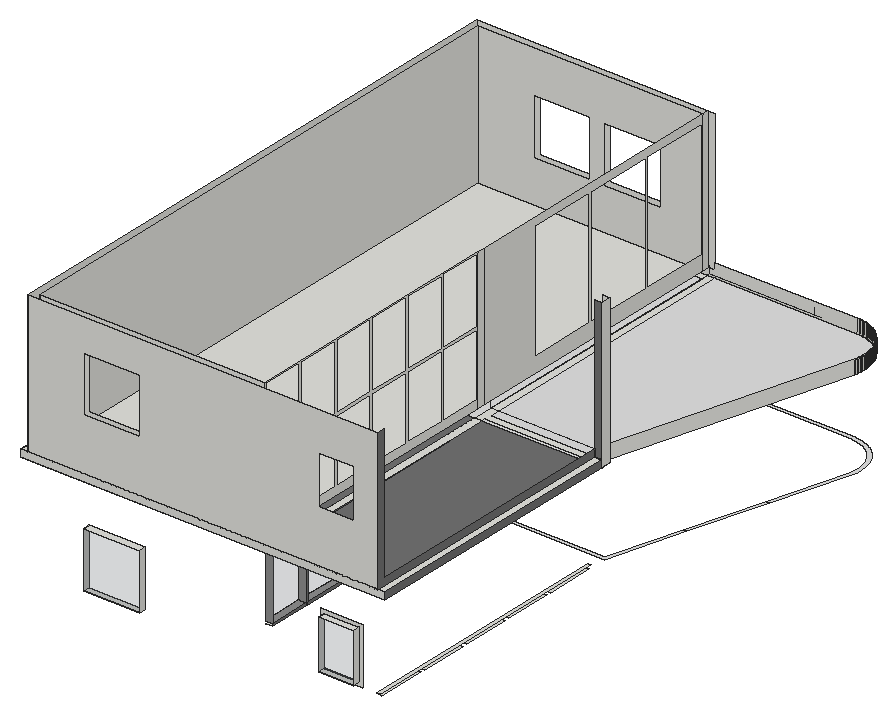
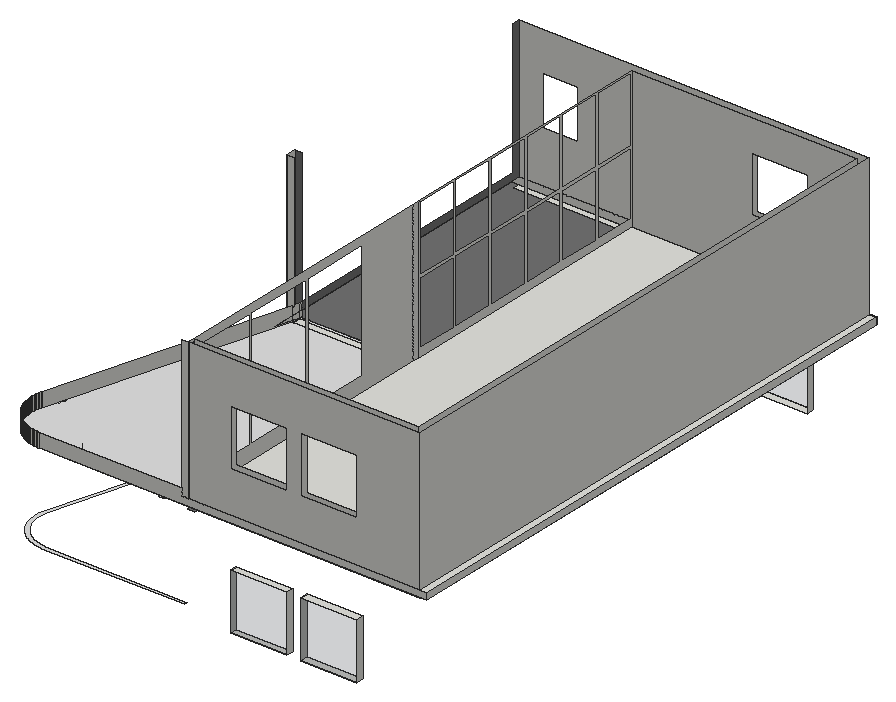
# SketchUp Ruby script. Lengths in inches.
U = 1.inch
M = Sketchup.active_model
def pt(a) = Geom::Point3d.new(a.map { |v| v * U })
def face(e, loops, mat)
  f = e.add_face(loops[0].map { |a| pt(a) })
  loops[1..].each { |l| e.add_face(l.map { |a| pt(a) }).erase! }
  f.material = f.back_material = mat if mat
  f
end
# faces: each face lists its corners as indices into pts; further lists are holes
def faces(e, pts, list, mat = nil) = list.each { |f| face(e, (f[0].is_a?(Array) ? f : [f]).map { |l| l.map { |i| pts[i] } }, mat) }
# xy, xz, yz: faces in a plane at the given z, y or x. An outline is a flat list of corners, or four numbers for a rectangle; further outlines are holes
def ring(l) = l.size == 4 ? [[l[0], l[1]], [l[2], l[1]], [l[2], l[3]], [l[0], l[3]]] : l.each_slice(2).to_a
def flat(e, list, mat, &to3) = list.each { |f| face(e, (f[0].is_a?(Array) ? f : [f]).map { |l| ring(l).map { |u, v| to3.(u, v) } }, mat) }
def xy(e, z, list, mat = nil) = flat(e, list, mat) { |x, y| [x, y, z] }
def xz(e, y, list, mat = nil) = flat(e, list, mat) { |x, z| [x, y, z] }
def yz(e, x, list, mat = nil) = flat(e, list, mat) { |y, z| [x, y, z] }
def lines(e, pts, list) = list.each { |a, b| e.add_line(pt(pts[a]), pt(pts[b])) }
# prism: a flat outline (further loops are holes) pulled along v
def prism(e, loops, v, mat = nil)
  f = face(e, loops, mat); d = Geom::Vector3d.new(v.map { |x| x * U })
  f.pushpull(f.normal.samedirection?(d) ? d.length : -d.length)
end
def box(e, o, s, mat = nil) = prism(e, [[o, [o[0] + s[0], o[1], o[2]], [o[0] + s[0], o[1] + s[1], o[2]], [o[0], o[1] + s[1], o[2]]]], [0, 0, s[2]], mat)
def at(x, y, z, deg = 0) = Geom::Transformation.translation(pt([x, y, z])) * Geom::Transformation.rotation(ORIGIN, Z_AXIS, deg.degrees)
def axes(o, x, y, z) = Geom::Transformation.new([*x, 0, *y, 0, *z, 0, *pt(o).to_a, 1])
def part(name) = M.definitions.add(name)
# library, detail: a bought-in or finely detailed component or shape, given as its bounding box
def library(name, o, s) = part(name).tap { |d| box(d.entities, o, s) }
def detail(e, o, s) = box(e.add_group.entities, o, s)
def put(e, d, t, mat = nil) = e.add_instance(d, t).tap { |i| i.material = mat if mat }
def group(e, t, mat = nil) = e.add_group.tap { |g| g.transformation = t; g.material = mat if mat }.entities
root = M.entities
M.materials.add("Glass_Basic_01").color = [105, 113, 122]
M.materials["Glass_Basic_01"].alpha = 0.25
M.materials.add("M01_Silver_Fog").color = [224, 224, 224]
M.materials.add("M04_Stone_Frost").color = [142, 142, 142]
M.materials.add("M06_Steel_Smoke").color = [114, 114, 114]
xy(root,300,[[54,0,102,6],[60,474,108,480],[120,474,168,480]])
xy(root,304,[[300,8,303,49],[300,53,303,94],[300,98,303,139],[300,143,303,184],[300,188,303,229]])
xy(root,306,[[300,6,303,231]])
xy(root,306,[[213,243,305.51,243,324.34,307.35,321.22,307.35,306,255.36,303.26,246,216,246,216,287.79,213,287.79],[321.22,307.35,324.34,307.35,343.2,371.78,340.07,371.78],[340.07,371.78,343.2,371.78,362.06,436.22,362.32,437.22,362.58,438.42,362.79,439.63,362.96,440.85,363.08,442.08,363.16,443.31,363.1875,444.54,363.17,445.77,363.1,447,362.99,448.22,362.83,449.44,362.63,450.66,362.38,451.86,362.08,453.06,361.74,454.24,361.35,455.41,360.92,456.5625,360.45,457.7,359.93,458.82,359.37,459.91,358.77,460.99,358.13,462.03,358.13,462.04,357.45,463.0625,356.73,464.0625,355.97,465.03,355.18,465.98,355.17,465.98,354.35,466.89,353.49,467.76,352.59,468.61,351.67,469.42,350.71,470.19,349.72,470.93,348.71,471.63,347.67,472.29,346.61,472.91,345.52,473.49,344.41,474.03,343.29,474.52,342.14,474.97,340.98,475.38,339.8,475.75,338.61,476.0625,337.41,476.34,336.2,476.5625,334.99,476.74,333.76,476.88,332.53,476.97,331.5,477,210,477,210,474,331.45,474,332.38,473.97,333.49,473.89,334.6,473.77,335.71,473.6,336.8,473.4,337.89,473.15,338.97,472.86,340.04,472.53,341.09,472.16,342.13,471.75,343.16,471.3,344.16,470.82,345.15,470.29,346.11,469.73,347.05,469.13,347.97,468.5,348.87,467.83,349.74,467.125,350.58,466.39,351.39,465.62,352.17,464.83,352.92,464,353.64,463.14,354.33,462.26,354.98,461.36,355.6,460.43,356.18,459.47,356.73,458.5,357.23,457.5,357.7,456.49,358.13,455.46,358.52,454.41,358.875,453.35,359.18,452.28,359.45,451.2,359.68,450.1,359.87,449,360.01,447.89,360.11,446.78,360.17,445.67,360.1875,444.55,360.16,443.43,360.09,442.32,359.98,441.21,359.83,440.1,359.63,439,359.4,437.91,359.17,437.01]],"M01_Silver_Fog")
xy(root,309,[[255,0,285,6]])
xy(root,325,[[204,7,210,43],[204,45,210,81],[204,83,210,119],[204,121,210,157],[204,159,210,195],
  [204,197,210,233]])
xy(root,327,[[204,7,210,43],[204,45,210,81],[204,83,210,119],[204,121,210,157],[204,159,210,195],
  [204,197,210,233]],"M04_Stone_Frost")
xy(root,348,[[54,0,102,6],[60,474,108,480],[120,474,168,480]])
xy(root,351,[[255,0,285,6]])
xy(root,377,[[204,295,210,353],[204,355,210,413],[204,415,210,473]],"M06_Steel_Smoke")
xy(root,383,[[204,7,210,43],[204,45,210,81],[204,83,210,119],[204,121,210,157],[204,159,210,195],
  [204,197,210,233]])
xy(root,383.24,[[225.03,477.03,225.29,477.03,225.38,477.04,225.46,477.06,225.55,477.08,225.71,477.14,225.87,477.22,225.95,477.27,226.02,477.32,226.08,477.38,226.15,477.4375,226.21,477.5,226.26,477.57,226.32,477.64,226.36,477.72,226.4,477.79,226.44,477.875,226.47,477.96,226.5,478.04,226.54,478.21,226.55,478.3,226.55,478.5625,226.54,478.65,226.52,478.74,226.5,478.82,226.47,478.9,226.4375,478.99,226.4,479.07,226.36,479.14,226.3125,479.22,226.26,479.29,226.2,479.35,226.14,479.42,226.08,479.48,226.01,479.53,225.9375,479.59,225.86,479.63,225.79,479.68,225.71,479.71,225.54,479.77,225.46,479.79,225.37,479.81,225.19,479.83,225.11,479.82,225.02,479.82,224.93,479.81,224.85,479.79,224.76,479.77,224.6,479.71,224.52,479.67,224.4375,479.63,224.36,479.58,224.29,479.53,224.23,479.47,224.16,479.41,224.1,479.35,224.05,479.28,223.99,479.21,223.95,479.13,223.91,479.06,223.87,478.98,223.84,478.9,223.81,478.8125,223.79,478.73,223.77,478.64,223.76,478.55,223.76,478.29,223.77,478.2,223.8125,478.03,223.84,477.95,223.87,477.87,223.95,477.71,224,477.64,224.05,477.56,224.11,477.5,224.17,477.43,224.23,477.37,224.37,477.27,224.45,477.22,224.52,477.18,224.6,477.14,224.68,477.11,224.77,477.08,224.85,477.06,224.94,477.04],[228.34,477.03,228.6,477.03,228.69,477.04,228.78,477.06,228.86,477.08,228.95,477.11,229.03,477.14,229.11,477.18,229.18,477.22,229.26,477.27,229.33,477.32,229.4,477.38,229.46,477.4375,229.52,477.5,229.58,477.57,229.63,477.64,229.67,477.72,229.72,477.79,229.75,477.875,229.79,477.96,229.8125,478.04,229.83,478.125,229.85,478.21,229.87,478.39,229.87,478.47,229.86,478.5625,229.85,478.65,229.83,478.74,229.81,478.82,229.78,478.9,229.75,478.99,229.71,479.07,229.67,479.14,229.62,479.22,229.57,479.29,229.51,479.35,229.45,479.42,229.39,479.48,229.32,479.53,229.25,479.59,229.18,479.63,229.1,479.68,229.02,479.71,228.9375,479.74,228.85,479.77,228.77,479.79,228.68,479.81,228.59,479.82,228.51,479.83,228.42,479.82,228.33,479.82,228.24,479.81,228.16,479.79,228.07,479.77,227.91,479.71,227.75,479.63,227.61,479.53,227.47,479.41,227.41,479.35,227.31,479.21,227.26,479.13,227.22,479.06,227.18,478.98,227.15,478.9,227.12,478.8125,227.1,478.73,227.08,478.64,227.07,478.55,227.07,478.29,227.09,478.2,227.1,478.12,227.125,478.03,227.15,477.95,227.18,477.87,227.26,477.71,227.3125,477.64,227.36,477.56,227.42,477.5,227.48,477.43,227.54,477.37,227.68,477.27,227.76,477.22,227.84,477.18,227.91,477.14,228,477.11,228.08,477.08,228.17,477.06,228.25,477.04]],"M01_Silver_Fog")
xy(root,384,[[0,0,6,231],[6,0,306,0,306,6,210,6,210,231,204,231,204,6,12,6,12,231,6,231],[0,231,6,480],[6,231,6,480,204,480,204,474,12,474,12,231],[204,231,210,231,210,234,306,234,306,240,210,240,210,480,204,480],
  [300,231,306,234],[306,231,306,234,307.76,240,312,240,312,231]])
xy(root,384,[[12,231,204,474],[210,231,300,234],[[306,234,306,240,210,240,210,480,331.55,480,332.69,479.96,334.03,479.87,335.37,479.72,336.7,479.52,338.02,479.28,339.33,478.98,340.63,478.63,341.92,478.23,343.1875,477.79,344.44,477.29,345.67,476.75,346.88,476.16,348.07,475.53,349.23,474.85,350.37,474.13,351.47,473.37,352.55,472.5625,353.6,471.72,354.61,470.83,355.59,469.91,356.53,468.95,357.39,468,357.4375,467.95,358.3,466.92,359.13,465.86,359.92,464.77,360.66,463.65,360.69,463.59,361.36,462.5,362.02,461.33,362.63,460.13,363.2,458.91,363.71,457.67,364.18,456.41,364.61,455.13,364.98,453.84,365.3,452.53,365.58,451.21,365.8,449.89,365.98,448.55,366.1,447.21,366.17,445.87,366.1875,444.52,366.16,443.18,366.07,441.84,365.94,440.5,365.76,439.16,365.52,437.84,365.24,436.52,364.95,435.42,307.76,240],[358.91,418.8,359,418.81,359.09,418.8125,359.17,418.83,359.26,418.85,359.34,418.87,359.43,418.9,359.51,418.9375,359.58,418.98,359.66,419.02,359.73,419.07,359.87,419.18,359.93,419.24,359.99,419.31,360.09,419.45,360.14,419.53,360.18,419.61,360.21,419.6875,360.24,419.77,360.27,419.85,360.29,419.94,360.3,420.03,360.31,420.11,360.31,420.29,360.3,420.38,360.29,420.46,360.27,420.55,360.24,420.64,360.18,420.8,360.14,420.88,360.09,420.95,360.04,421.03,359.99,421.09,359.93,421.16,359.87,421.22,359.73,421.34,359.66,421.38,359.58,421.43,359.51,421.47,359.43,421.5,359.34,421.53,359.26,421.56,359.17,421.58,359.09,421.59,359,421.6,358.82,421.6,358.73,421.59,358.65,421.58,358.5625,421.56,358.48,421.53,358.39,421.5,358.3125,421.47,358.24,421.43,358.16,421.38,358.09,421.34,357.95,421.22,357.89,421.16,357.83,421.09,357.78,421.03,357.73,420.95,357.68,420.88,357.64,420.8,357.58,420.64,357.55,420.55,357.54,420.46,357.52,420.38,357.51,420.29,357.51,420.11,357.52,420.03,357.54,419.94,357.55,419.85,357.58,419.77,357.61,419.6875,357.64,419.61,357.68,419.53,357.73,419.45,357.83,419.31,357.89,419.24,357.95,419.18,358.09,419.07,358.16,419.02,358.24,418.98,358.3125,418.9375,358.39,418.9,358.48,418.87,358.5625,418.85,358.65,418.83,358.73,418.8125,358.82,418.81],[359.74,421.95,359.92,421.95,360.01,421.96,360.09,421.97,360.18,421.99,360.26,422.02,360.35,422.05,360.43,422.08,360.51,422.12,360.58,422.17,360.65,422.21,360.79,422.33,360.91,422.45,360.96,422.52,361.01,422.6,361.06,422.67,361.1,422.75,361.16,422.91,361.1875,423,361.21,423.08,361.23,423.26,361.23,423.44,361.22,423.52,361.21,423.61,361.1875,423.7,361.16,423.78,361.1,423.94,361.06,424.02,361.01,424.1,360.91,424.24,360.85,424.31,360.79,424.37,360.72,424.43,360.58,424.53,360.51,424.57,360.35,424.65,360.26,424.68,360.18,424.7,360.09,424.72,360.01,424.74,359.92,424.74,359.83,424.75,359.74,424.74,359.66,424.74,359.48,424.7,359.4,424.68,359.32,424.65,359.23,424.61,359.16,424.57,359.08,424.53,359.01,424.48,358.9375,424.43,358.87,424.37,358.81,424.31,358.75,424.24,358.65,424.1,358.6,424.02,358.5625,423.94,358.53,423.86,358.47,423.7,358.46,423.61,358.44,423.52,358.43,423.44,358.43,423.26,358.44,423.17,358.46,423.08,358.47,423,358.5,422.91,358.53,422.83,358.5625,422.75,358.6,422.67,358.65,422.6,358.7,422.52,358.75,422.45,358.87,422.33,358.9375,422.27,359.01,422.21,359.08,422.17,359.16,422.12,359.23,422.08,359.32,422.05,359.48,421.99,359.57,421.97,359.66,421.96]],[358.91,418.8,359,418.81,359.09,418.8125,359.17,418.83,359.26,418.85,359.34,418.87,359.43,418.9,359.51,418.9375,359.58,418.98,359.66,419.02,359.73,419.07,359.87,419.18,359.93,419.24,359.99,419.31,360.09,419.45,360.14,419.53,360.18,419.61,360.21,419.6875,360.24,419.77,360.27,419.85,360.29,419.94,360.3,420.03,360.31,420.11,360.31,420.29,360.3,420.38,360.29,420.46,360.27,420.55,360.24,420.64,360.18,420.8,360.14,420.88,360.09,420.95,360.04,421.03,359.99,421.09,359.93,421.16,359.87,421.22,359.73,421.34,359.66,421.38,359.58,421.43,359.51,421.47,359.43,421.5,359.34,421.53,359.26,421.56,359.17,421.58,359.09,421.59,359,421.6,358.82,421.6,358.73,421.59,358.65,421.58,358.5625,421.56,358.48,421.53,358.39,421.5,358.3125,421.47,358.24,421.43,358.16,421.38,358.09,421.34,357.95,421.22,357.89,421.16,357.83,421.09,357.78,421.03,357.73,420.95,357.68,420.88,357.64,420.8,357.58,420.64,357.55,420.55,357.54,420.46,357.52,420.38,357.51,420.29,357.51,420.11,357.52,420.03,357.54,419.94,357.55,419.85,357.58,419.77,357.61,419.6875,357.64,419.61,357.68,419.53,357.73,419.45,357.83,419.31,357.89,419.24,357.95,419.18,358.09,419.07,358.16,419.02,358.24,418.98,358.3125,418.9375,358.39,418.9,358.48,418.87,358.5625,418.85,358.65,418.83,358.73,418.8125,358.82,418.81],[359.74,421.95,359.92,421.95,360.01,421.96,360.09,421.97,360.18,421.99,360.26,422.02,360.35,422.05,360.43,422.08,360.51,422.12,360.58,422.17,360.65,422.21,360.79,422.33,360.91,422.45,360.96,422.52,361.01,422.6,361.06,422.67,361.1,422.75,361.16,422.91,361.1875,423,361.21,423.08,361.23,423.26,361.23,423.44,361.22,423.52,361.21,423.61,361.1875,423.7,361.16,423.78,361.1,423.94,361.06,424.02,361.01,424.1,360.91,424.24,360.85,424.31,360.79,424.37,360.72,424.43,360.58,424.53,360.51,424.57,360.35,424.65,360.26,424.68,360.18,424.7,360.09,424.72,360.01,424.74,359.92,424.74,359.83,424.75,359.74,424.74,359.66,424.74,359.48,424.7,359.4,424.68,359.32,424.65,359.23,424.61,359.16,424.57,359.08,424.53,359.01,424.48,358.9375,424.43,358.87,424.37,358.81,424.31,358.75,424.24,358.65,424.1,358.6,424.02,358.5625,423.94,358.53,423.86,358.47,423.7,358.46,423.61,358.44,423.52,358.43,423.44,358.43,423.26,358.44,423.17,358.46,423.08,358.47,423,358.5,422.91,358.53,422.83,358.5625,422.75,358.6,422.67,358.65,422.6,358.7,422.52,358.75,422.45,358.87,422.33,358.9375,422.27,359.01,422.21,359.08,422.17,359.16,422.12,359.23,422.08,359.32,422.05,359.48,421.99,359.57,421.97,359.66,421.96]],"M01_Silver_Fog")
xy(root,384,[[306,0,306,6,210,6,210,231,312,231,312,0],[12,6,204,231]],"M06_Steel_Smoke")
xy(root,384.01,[[306,231,312,240]])
xy(root,390,[[0,0,6,480],[306,0,312,231],[12,6,204,474]])
xz(root,0,[[0,384,312,390],[[6,390,306,510],[54,435,102,483],[255,435,285,477]]])
xz(root,0,[[54,300,102,348],[255,309,285,351]],"Glass_Basic_01")
xz(root,6,[[[252,306,288,354],[255,309,285,351]],[[12,390,204,510],[54,435,102,483]]])
xz(root,7,[[204,327,210,383]],"M04_Stone_Frost")
xz(root,43,[[204,327,210,383]],"M04_Stone_Frost")
xz(root,45,[[204,327,210,383]],"M04_Stone_Frost")
xz(root,81,[[204,327,210,383]],"M04_Stone_Frost")
xz(root,83,[[204,327,210,383]],"M04_Stone_Frost")
xz(root,119,[[204,327,210,383]],"M04_Stone_Frost")
xz(root,121,[[204,327,210,383]],"M04_Stone_Frost")
xz(root,157,[[204,327,210,383]],"M04_Stone_Frost")
xz(root,159,[[204,327,210,383]],"M04_Stone_Frost")
xz(root,195,[[204,327,210,383]],"M04_Stone_Frost")
xz(root,197,[[204,327,210,383]],"M04_Stone_Frost")
xz(root,231,[[306,384.01,312,390]])
xz(root,231,[[306,384,312,384.01],[306,390,312,510]],"M06_Steel_Smoke")
xz(root,233,[[204,327,210,383]],"M04_Stone_Frost")
xz(root,240,[[307.76,384,312,384.01],[307.76,384.01,307.76,396,306,396,306,510.01,307.76,510.01,307.76,510,312,510,312,384.01]])
xz(root,474,[[[12,390,204,510],[120,426,168,474],[60,426,108,474]]])
xz(root,480,[[0,384,0,390,210,390,210,396,331.55,396,331.55,384],[[6,390,204,510],[60,426,108,474],[120,426,168,474]],[204,390,210,510]])
xz(root,480,[[60,300,108,348],[120,300,168,348]],"Glass_Basic_01")
yz(root,0,[[0,384,480,390]])
yz(root,6,[[0,390,480,510]])
yz(root,12,[[6,390,474,510]])
yz(root,54,[[0,300,6,348]])
yz(root,60,[[474,300,480,348]])
yz(root,102,[[0,300,6,348]])
yz(root,108,[[474,300,480,348]])
yz(root,120,[[474,300,480,348]])
yz(root,168,[[474,300,480,348]])
yz(root,204,[[[6,390,234,510],[7,453,43,509],[121,453,157,509],[159,453,195,509],[197,453,233,509],[45,453,81,509],[83,453,119,509],[7,397,43,451],[197,397,233,451],[159,397,195,451],[121,397,157,451],[45,397,81,451],[83,397,119,451]],[234,390,240,510],[[240,390,474,510],[415,403,473,503],[295,403,353,503],[355,403,413,503]],[474,390,480,510]])
yz(root,204,[[7,327,43,383],[45,327,81,383],[83,327,119,383],[121,327,157,383],[159,327,195,383],
  [197,327,233,383]],"Glass_Basic_01")
yz(root,210,[[286.46,316.46,288,337.54]])
yz(root,210,[[7,325,43,327],[45,325,81,327],[83,325,119,327],[121,325,157,327],[159,325,195,327],
  [197,325,233,327],[44,327,45,327,45,383,81,383,81,327,82,327,82,384,44,384],[82,327,83,327,83,383,119,383,119,327,120,327,120,384,82,384],[120,327,121,327,121,383,157,383,157,327,158,327,158,384,120,384],[158,327,159,327,159,383,195,383,195,327,196,327,196,384,158,384]],"M06_Steel_Smoke")
yz(root,255,[[0,309,6,351]])
yz(root,285,[[0,309,6,351]])
yz(root,306,[[231,384,234,384.01],[234,384,240,384.01],[231,384.01,234,390],[231,390,234,396]])
yz(root,306,[[0,390,231,390,231,396,6,396,6,510,0,510]],"M06_Steel_Smoke")
yz(root,312,[[231,384,240,384.01],[231,384.01,240,510]])
yz(root,312,[[0,384,231,390]],"M06_Steel_Smoke")
p = [[306,234,384],[307.76,240,384],[307.76,240,384.01],[307.76,240,396],[306,234,396],[306,234,390],
  [306,234,384.01],[364.95,435.42,396],[364.95,435.42,384],[365.24,436.52,396],[365.24,436.52,384],[365.52,437.84,396],
  [365.52,437.84,384],[365.76,439.16,396],[365.76,439.16,384],[365.94,440.5,396],[365.94,440.5,384],[366.07,441.84,396],
  [366.07,441.84,384],[366.16,443.18,396],[366.16,443.18,384],[366.1875,444.52,396],[366.1875,444.52,384],[366.17,445.87,396],
  [366.17,445.87,384],[366.1,447.21,396],[366.1,447.21,384],[365.98,448.55,396],[365.98,448.55,384],[365.8,449.89,396],
  [365.8,449.89,384],[365.58,451.21,396],[365.58,451.21,384],[365.3,452.53,396],[365.3,452.53,384],[364.98,453.84,396],
  [364.98,453.84,384],[364.61,455.13,396],[364.61,455.13,384],[364.18,456.41,396],[364.18,456.41,384],[363.71,457.67,396],
  [363.71,457.67,384],[363.2,458.91,396],[363.2,458.91,384],[362.63,460.13,396],[362.63,460.13,384],[362.02,461.33,396],
  [362.02,461.33,384],[361.36,462.5,396],[361.36,462.5,384],[360.69,463.59,396],[360.69,463.59,384],[359.92,464.77,396],
  [360.66,463.65,396],[360.66,463.65,384],[359.92,464.77,384],[359.13,465.86,396],[359.13,465.86,384],[358.3,466.92,396],
  [358.3,466.92,384],[357.4375,467.95,396],[357.4375,467.95,384],[356.53,468.95,396],[357.39,468,396],[357.39,468,384],
  [356.53,468.95,384],[355.59,469.91,396],[355.59,469.91,384],[354.61,470.83,396],[354.61,470.83,384],[353.6,471.72,396],
  [353.6,471.72,384],[352.55,472.5625,396],[352.55,472.5625,384],[351.47,473.37,396],[351.47,473.37,384],[350.37,474.13,396],
  [350.37,474.13,384],[349.23,474.85,396],[349.23,474.85,384],[348.07,475.53,396],[348.07,475.53,384],[346.88,476.16,396],
  [346.88,476.16,384],[345.67,476.75,396],[345.67,476.75,384],[344.44,477.29,396],[344.44,477.29,384],[343.1875,477.79,396],
  [343.1875,477.79,384],[341.92,478.23,396],[341.92,478.23,384],[340.63,478.63,396],[340.63,478.63,384],[339.33,478.98,396],
  [339.33,478.98,384],[338.02,479.28,396],[338.02,479.28,384],[336.7,479.52,396],[336.7,479.52,384],[335.37,479.72,396],
  [335.37,479.72,384],[334.03,479.87,396],[334.03,479.87,384],[332.69,479.96,396],[332.69,479.96,384],[331.55,480,396],
  [331.55,480,384],[306,260.5,390],[210,240,390],[210,474,390],[210,474,396],[300,474,390],
  [300,474,396],[210,240,396],[300,240,390],[306,474,390]]
faces(root,p,[[0,1,2,3,4,5,6],[7,3,2,1,8],[9,7,8,10],[11,9,10,12],[13,11,12,14],[15,13,14,16],[17,15,16,18],[19,17,18,20],
  [21,19,20,22],[23,21,22,24],[25,23,24,26],[27,25,26,28],[29,27,28,30],[31,29,30,32],[33,31,32,34],[35,33,34,36],
  [37,35,36,38],[39,37,38,40],[41,39,40,42],[43,41,42,44],[45,43,44,46],[47,45,46,48],[49,47,48,50],[51,49,50,52],
  [53,54,55,56],[54,51,52,55],[57,53,56,58],[59,57,58,60],[61,59,60,62],[63,64,65,66],[64,61,62,65],[67,63,66,68],
  [69,67,68,70],[71,69,70,72],[73,71,72,74],[75,73,74,76],[77,75,76,78],[79,77,78,80],[81,79,80,82],[83,81,82,84],
  [85,83,84,86],[87,85,86,88],[89,87,88,90],[91,89,90,92],[93,91,92,94],[95,93,94,96],[97,95,96,98],[99,97,98,100],
  [101,99,100,102],[103,101,102,104],[105,103,104,106],[107,105,106,108]])
lines(root,p,[[109,5],[110,111],[111,112],[113,114],[110,115],[116,110],[113,111],[113,117],[116,109]])
